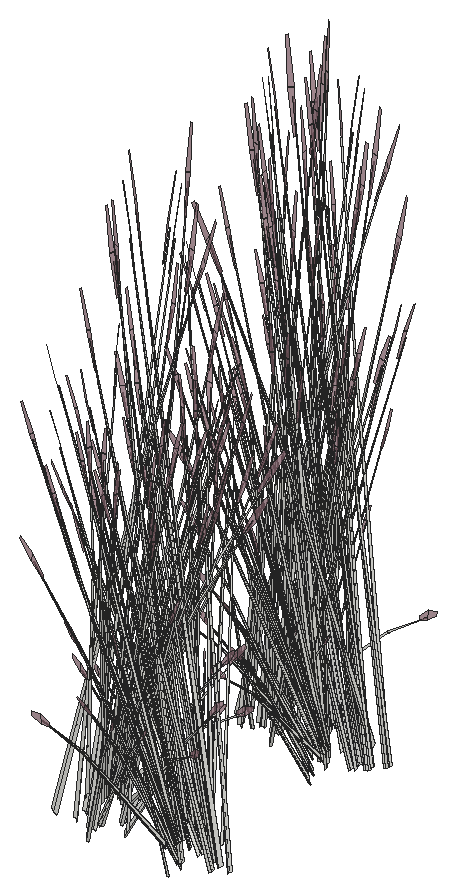
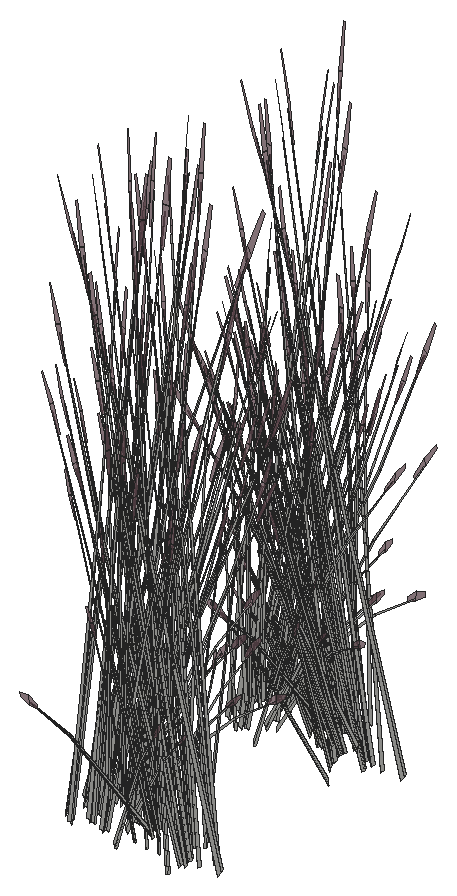
# SketchUp Ruby script. Lengths in inches.
U = 1.inch
M = Sketchup.active_model
def pt(a) = Geom::Point3d.new(a.map { |v| v * U })
def face(e, loops, mat)
  f = e.add_face(loops[0].map { |a| pt(a) })
  loops[1..].each { |l| e.add_face(l.map { |a| pt(a) }).erase! }
  f.material = f.back_material = mat if mat
  f
end
# faces: each face lists its corners as indices into pts; further lists are holes
def faces(e, pts, list, mat = nil) = list.each { |f| face(e, (f[0].is_a?(Array) ? f : [f]).map { |l| l.map { |i| pts[i] } }, mat) }
# xy, xz, yz: faces in a plane at the given z, y or x. An outline is a flat list of corners, or four numbers for a rectangle; further outlines are holes
def ring(l) = l.size == 4 ? [[l[0], l[1]], [l[2], l[1]], [l[2], l[3]], [l[0], l[3]]] : l.each_slice(2).to_a
def flat(e, list, mat, &to3) = list.each { |f| face(e, (f[0].is_a?(Array) ? f : [f]).map { |l| ring(l).map { |u, v| to3.(u, v) } }, mat) }
def xy(e, z, list, mat = nil) = flat(e, list, mat) { |x, y| [x, y, z] }
def xz(e, y, list, mat = nil) = flat(e, list, mat) { |x, z| [x, y, z] }
def yz(e, x, list, mat = nil) = flat(e, list, mat) { |y, z| [x, y, z] }
def lines(e, pts, list) = list.each { |a, b| e.add_line(pt(pts[a]), pt(pts[b])) }
# prism: a flat outline (further loops are holes) pulled along v
def prism(e, loops, v, mat = nil)
  f = face(e, loops, mat); d = Geom::Vector3d.new(v.map { |x| x * U })
  f.pushpull(f.normal.samedirection?(d) ? d.length : -d.length)
end
def box(e, o, s, mat = nil) = prism(e, [[o, [o[0] + s[0], o[1], o[2]], [o[0] + s[0], o[1] + s[1], o[2]], [o[0], o[1] + s[1], o[2]]]], [0, 0, s[2]], mat)
def at(x, y, z, deg = 0) = Geom::Transformation.translation(pt([x, y, z])) * Geom::Transformation.rotation(ORIGIN, Z_AXIS, deg.degrees)
def axes(o, x, y, z) = Geom::Transformation.new([*x, 0, *y, 0, *z, 0, *pt(o).to_a, 1])
def part(name) = M.definitions.add(name)
# library, detail: a bought-in or finely detailed component or shape, given as its bounding box
def library(name, o, s) = part(name).tap { |d| box(d.entities, o, s) }
def detail(e, o, s) = box(e.add_group.entities, o, s)
def put(e, d, t, mat = nil) = e.add_instance(d, t).tap { |i| i.material = mat if mat }
def group(e, t, mat = nil) = e.add_group.tap { |g| g.transformation = t; g.material = mat if mat }.entities
root = M.entities
M.materials.add("LightPink_Translucent").color = [144, 107, 117]
M.materials["LightPink_Translucent"].alpha = 0.75
c1 = part("blade")
p = [[2.15,0.21,22],[0,0.17,0],[0.09,0.45,0],[2.18,0.31,22],[2.29,0.31,22],[0.38,0.45,0],
  [2.48,0.24,33],[2.49,0.24,33],[2.48,0.22,33]]
faces(c1.entities,p,[[0,1,2,3],[4,5,2,3],[6,3,4,7],[8,0,3,6]])
c2 = part("seeds")
p = [[0.3,-0.1,1.38],[-0.01,-0.03,1.59],[-0.01,-0.03,0.03],[0.14,-0.07,-0.07],[0.29,-0.03,3],[0.15,0.01,3.11]]
faces(c2.entities,p,[[0,1,2,3],[1,0,4,5]],"LightPink_Translucent")
c3 = part("blade with seeds")
put(c3.entities,c1,at(0,0,0))
put(c3.entities,c2,axes([2.4,0.25,30.99],[1.5799,-0.05474,1.17369],[-0.12525,1.92788,0.29478],[-0.07173,-0.02425,1.56792]))
put(root,c3,axes([504.82,142.39,3.91],[-0.16348,-0.00431,1.74944],[-0.52047,0.43131,-0.27667],[-0.2777,-0.08813,0.14031]))
put(root,c3,axes([506.71,143.05,4.24],[0.11735,0.49217,0.35414],[-0.67083,0.12996,-0.4572],[-0.18018,-0.14104,0.87481]))
put(root,c3,axes([504.7,143.37,4.29],[0.62747,-0.45094,0.53763],[0.54116,0.47889,0.4433],[-0.29439,-0.08318,1.11249]))
put(root,c3,axes([495.97,144.28,0.6875],[-0.11372,-0.04814,1.76342],[-0.29211,-0.53779,-0.26939],[0.19706,-0.14594,0.30037]))
put(root,c3,axes([495.33,144.6,3.93],[0.54105,0.41691,0.48003],[-0.57458,0.35956,0.3958],[0.0998,-0.1956,0.9933]))
put(root,c3,axes([504.98,143.37,3.92],[0.03826,-0.46465,0.0643],[0.57772,0.01274,0.50621],[-0.2213,-0.04862,0.77189]))
put(root,c3,axes([504.76,143.51,3.72],[-0.43232,-0.38257,-0.35414],[0.49364,-0.36215,0.4572],[-0.25081,-0.0551,0.87481]))
put(root,c3,axes([495.97,145.8,4.17],[0.39688,-0.48213,-0.71045],[0.69548,0.34264,0.08574],[0.23697,-0.17468,1.00501]))
put(root,c3,axes([495.95,145.57,3.875],[-0.19519,-0.55794,-0.51099],[0.73919,-0.0976,-0.3958],[0.21183,-0.14986,0.97773]))
put(root,c3,axes([504.81,142.86,1.32],[-0.21918,0.49894,-0.03893],[-0.6746,-0.15348,-0.17649],[-0.10242,-0.08161,0.58215]))
put(root,c3,axes([504.45,145.14,1.57],[-0.95008,0,0],[0,-0.68292,-0.51607],[0,-0.15554,1.63711]))
put(root,c3,axes([504.61,143.92,1.78],[0.14835,0.17012,1.43002],[-0.34183,0.46242,-0.30754],[-0.351,-0.11053,0.61141]))
put(root,c3,axes([496.3,145.97,4.23],[-0.70283,-0.33692,-0.1216],[0.40491,-0.48793,-0.67495],[0.19857,-0.16961,1.02557]))
put(root,c3,axes([505.22,143.77,4.17],[-0.75952,-0.01471,-0.71045],[0.05101,-0.61953,0.08574],[-0.32177,-0.06538,1.00501]))
put(root,c3,axes([496.55,145.35,1.78],[-0.27143,-0.0181,1.43002],[-0.27808,-0.48551,-0.30754],[0.33346,-0.13735,0.61141]))
put(root,c3,axes([498.03,145.82,3.9],[-0.09924,-0.00464,1.77383],[-0.4121,-0.49725,-0.16761],[0.1655,-0.1635,0.31391]))
put(root,c3,axes([493.17,145.55,1.25],[0.51177,-0.45928,-0.62353],[0.63575,0.41646,-0.16365],[0.20507,-0.11457,1.37633]))
put(root,c3,axes([496.86,144.46,1.96],[-0.25308,0.31105,1.1486],[-0.21753,-0.4179,0.84392],[0.20902,-0.10472,0.25299]))
put(root,c3,axes([504.1875,142.76,3.9],[0.05633,0.06098,1.77383],[-0.27155,0.54815,-0.16761],[-0.27501,0.00397,0.31391]))
put(root,c3,axes([496.5,145.63,3.72],[0.66138,-0.08733,-0.35414],[0.17464,0.49921,0.4572],[0.18953,-0.13408,0.87481]))
put(root,c3,axes([504.97,143.89,3.875],[-0.55171,0.40476,-0.51099],[-0.48318,-0.42758,-0.3958],[-0.28031,-0.06159,0.97773]))
put(root,c3,axes([505.375,143.71,4.24],[0.43232,0.38257,0.35414],[-0.49364,0.36215,-0.4572],[-0.25081,-0.0551,0.87481]))
put(root,c3,axes([503.72,144.43,1.96],[0.48508,-0.04372,1.1486],[-0.3077,0.38525,0.84392],[-0.23971,-0.05779,0.25299]))
put(root,c3,axes([495.96,145.92,4.24],[-0.66138,0.08733,0.35414],[-0.17464,-0.49921,-0.4572],[0.18953,-0.13408,0.87481]))
put(root,c3,axes([505.26,143.47,4.23],[-0.04068,0.62141,-0.1216],[-0.77029,-0.01698,-0.67495],[-0.29667,-0.04317,1.02557]))
put(root,c3,axes([496.56,145.85,3.92],[0.52161,0.25698,0.0643],[-0.30368,0.36595,0.50621],[0.16723,-0.11831,0.77189]))
put(root,c3,axes([496.41,145.74,3.93],[0.18844,0.56237,0.48003],[-0.73919,0.0976,0.3958],[0.21785,-0.13226,0.9933]))
put(root,c3,axes([498.4,146.42,3.91],[0.10543,-0.09307,1.74944],[-0.13495,-0.57092,-0.27667],[0.26455,-0.10825,0.14031]))
put(root,c3,axes([506.62,145.93,1.25],[-0.79037,-0.10018,-0.62353],[0.16679,-0.61794,-0.16365],[-0.23587,-0.07488,1.37633]))
put(root,c3,axes([504.15,144.78,3.93],[0.21466,-0.55714,0.48003],[0.70573,0.19051,0.3958],[-0.27753,0.03348,0.9933]))
put(root,c3,axes([504.09,144.63,3.92],[-0.27906,-0.41663,0.0643],[0.50888,-0.20393,0.50621],[-0.22432,0.04024,0.77189]))
put(root,c3,axes([504.08,145.06,0.6875],[0.01927,0.0963,1.76342],[-0.38846,0.5029,-0.26939],[-0.27592,-0.02535,0.30037]))
put(root,c3,axes([505.78,146.875,1.22],[-0.17848,-0.53243,-0.30978],[0.70886,-0.15119,0.30978],[-0.1429,-0.0614,1.38974]))
put(root,c3,axes([496.33,147.29,4.23],[-0.38229,-0.5533,-0.1216],[0.6785,-0.2719,-0.67495],[0.28593,-0.073,1.02557]))
put(root,c3,axes([496.29,146.81,3.875],[0.20584,-0.55581,-0.51099],[0.70573,0.19051,-0.3958],[0.28414,-0.05097,0.97773]))
put(root,c3,axes([495.18,144.55,1.57],[0.47504,-0.61229,0],[0.79476,0.34146,-0.51607],[0.18101,0.07777,1.63711]))
put(root,c3,axes([505.58,147.1,1.21],[-0.7111,-0.30552,-0.49651],[0.42504,-0.54784,0],[-0.16196,-0.06958,1.57504]))
put(root,c3,axes([504,144.84,3.72],[-0.63144,-0.17046,-0.35414],[0.18417,-0.49731,0.4572],[-0.25423,0.0456,0.87481]))
put(root,c3,axes([497.05,146.97,1.17],[-0.48937,0.07333,1.41583],[-0.07789,-0.58369,0.08104],[0.34275,-0.08835,0.80566]))
put(root,c3,axes([497.9375,146.45,1.45],[-0.47106,-0.39072,-0.06488],[0.51591,-0.35801,-0.29416],[0.14618,-0.02521,0.97024]))
put(root,c3,axes([507.52,146.02,1.86],[-0.76714,0.40567,-0.29095],[-0.51013,-0.57321,-0.50002],[-0.18927,-0.05821,1.59708]))
put(root,c3,axes([496.16,147.01,4.17],[0.66765,-0.26986,-0.71045],[0.37208,0.55551,0.08574],[0.32259,-0.0631,1.00501]))
put(root,c3,axes([496.0625,147.12,4.24],[-0.63144,-0.17046,0.35414],[0.18417,-0.49731,-0.4572],[0.25423,-0.0456,0.87481]))
put(root,c3,axes([504.67,144.79,4.24],[0.63144,0.17046,0.35414],[-0.18417,0.49731,-0.4572],[-0.25423,0.0456,0.87481]))
put(root,c3,axes([491.74,145.63,0.79],[-0.74787,0.24464,1.28929],[-0.23804,-0.70192,0.50096],[0.45924,0.01168,1.46642]))
put(root,c3,axes([497.58,146.59,0.6875],[-0.03971,-0.09277,1.76342],[0.27541,-0.54264,-0.26939],[0.27782,-0.00781,0.30037]))
put(root,c3,axes([505.92,144.76,2.53],[0.21597,-0.08839,1.77064],[0.07448,0.61717,0.13857],[-0.4678,0.08189,0.63284]))
put(root,c3,axes([493.68,145.99,1.86],[0.76714,-0.40567,-0.29095],[0.51013,0.57321,-0.50002],[0.18927,0.05821,1.59708]))
put(root,c3,axes([496.73,147.0625,3.72],[0.63144,0.17046,-0.35414],[-0.18417,0.49731,0.4572],[0.25423,-0.0456,0.87481]))
put(root,c3,axes([495.61,144.92,1.21],[0.7111,0.30552,-0.49651],[-0.42504,0.54784,0],[0.16196,0.06958,1.57504]))
put(root,c3,axes([503.6,145.17,3.91],[-0.12407,0.07933,1.74944],[0.01055,0.57963,-0.27667],[-0.2844,0.07538,0.14031]))
put(root,c3,axes([504.43,145.09,3.875],[-0.20584,0.55581,-0.51099],[-0.70573,-0.19051,-0.3958],[-0.28414,0.05097,0.97773]))
put(root,c3,axes([504.4,144.62,4.23],[0.38229,0.5533,-0.1216],[-0.6785,0.2719,-0.67495],[-0.28593,0.073,1.02557]))
put(root,c3,axes([506.02,147.47,1.57],[-0.47504,0.61229,0],[-0.79476,-0.34146,-0.51607],[-0.18101,-0.07777,1.63711]))
put(root,c3,axes([495.01,146.45,3.07],[-0.31515,0.01384,1.71376],[0.20907,-0.5998,0.13857],[0.44912,0.0371,0.73262]))
put(root,c3,axes([495.41,145.14,1.22],[0.17848,0.53243,-0.30978],[-0.70886,0.15119,0.30978],[0.1429,0.0614,1.38974]))
put(root,c3,axes([496.63,147.27,3.92],[0.27906,0.41663,0.0643],[-0.50888,0.20393,0.50621],[0.22432,-0.04024,0.77189]))
put(root,c3,axes([496.58,147.125,3.93],[-0.21466,0.55714,0.48003],[-0.70573,-0.19051,0.3958],[0.27753,-0.03348,0.9933]))
put(root,c3,axes([494.57,146.09,1.25],[0.79037,0.10018,-0.62353],[-0.16679,0.61794,-0.16365],[0.23587,0.07488,1.37633]))
put(root,c3,axes([504.32,146.17,3.93],[-0.18844,-0.56237,0.48003],[0.73919,-0.0976,0.3958],[-0.21785,0.13226,0.9933]))
put(root,c3,axes([498.07,147.16,1.96],[-0.46945,0.10088,1.1486],[0.22097,-0.4169,0.84392],[0.24904,0.02853,0.25299]))
put(root,c3,axes([504.17,146.06,3.92],[-0.52161,-0.25698,0.0643],[0.30368,-0.36595,0.50621],[-0.16723,0.11831,0.77189]))
put(root,c3,axes([497.85,148.93,3.9],[-0.0687,-0.05349,1.77383],[0.15029,-0.57341,-0.16761],[0.27062,-0.03664,0.31391]))
put(root,c3,axes([497.25,148.45,3.12],[-0.14542,-0.51365,-0.03492],[0.68734,-0.11809,-0.15832],[0.14353,0.03256,0.52218]))
put(root,c3,axes([495.47,148.44,4.23],[0.04068,-0.62141,-0.1216],[0.77029,0.01698,-0.67495],[0.29667,0.04317,1.02557]))
put(root,c3,axes([504.77,145.98,4.24],[0.66138,-0.08733,0.35414],[0.17464,0.49921,-0.4572],[-0.18953,0.13408,0.87481]))
put(root,c3,axes([502.22,145.76,3.9],[0.09697,0.01639,1.77383],[0.29997,0.53988,-0.16761],[-0.1985,0.1417,0.31391]))
put(root,c3,axes([495.35,148.19,4.24],[-0.43232,-0.38257,0.35414],[0.49364,-0.36215,-0.4572],[0.25081,0.0551,0.87481]))
put(root,c3,axes([503.04,147.47,1.96],[0.31665,-0.27694,1.1486],[0.12495,0.43841,0.84392],[-0.22883,0.0785,0.25299]))
put(root,c3,axes([504.23,146.28,3.72],[-0.66138,0.08733,-0.35414],[-0.17464,-0.49921,0.4572],[-0.18953,0.13408,0.87481]))
put(root,c3,axes([496.14,148.0625,3.91],[0.16299,-0.01033,1.74944],[0.44707,-0.47471,-0.27667],[0.28992,0.06266,0.14031]))
put(root,c3,axes([503.27,147.4,4.84],[0.67048,0.16311,-0.06488],[-0.20625,0.50201,-0.29416],[-0.10966,0.07622,0.97024]))
put(root,c3,axes([508.03,146.47,1.25],[-0.51177,0.45928,-0.62353],[-0.63575,-0.41646,-0.16365],[-0.20507,0.11457,1.37633]))
put(root,c3,axes([495.51,148.14,4.17],[0.75952,0.01471,-0.71045],[-0.05101,0.61953,0.08574],[0.32177,0.06538,1.00501]))
put(root,c3,axes([504.43,145.93,4.23],[0.70283,0.33692,-0.1216],[-0.40491,0.48793,-0.67495],[-0.19857,0.16961,1.02557]))
put(root,c3,axes([505.375,145.78,3.07],[0.18977,-0.18775,1.71376],[0.47917,0.50677,0.13857],[-0.32866,0.23079,0.73262]))
put(root,c3,axes([496.75,146.88,1.57],[0.95008,0,0],[0,0.68292,-0.51607],[0,0.15554,1.63711]))
put(root,c3,axes([504.78,146.33,3.875],[0.19519,0.55794,-0.51099],[-0.73919,0.0976,-0.3958],[-0.21183,0.14986,0.97773]))
put(root,c3,axes([495.96,148.39,3.72],[0.43232,0.38257,-0.35414],[-0.49364,0.36215,0.4572],[0.25081,0.0551,0.87481]))
put(root,c3,axes([495.74,148.54,3.92],[-0.03826,0.46465,0.0643],[-0.57772,-0.01274,0.50621],[0.2213,0.04862,0.77189]))
put(root,c3,axes([505.2,147.27,3.92],[-0.62439,-0.02847,0.0643],[0.01712,-0.42991,0.50621],[-0.06534,0.16468,0.77189]))
put(root,c3,axes([503.87,147.76,0.6875],[0.10192,0.06105,1.76342],[0.17281,0.56562,-0.26939],[-0.22588,0.12062,0.30037]))
put(root,c3,axes([505.4,147.31,3.93],[-0.54105,-0.41691,0.48003],[0.57458,-0.35956,0.3958],[-0.0998,0.1956,0.9933]))
put(root,c3,axes([495.8,148.39,3.93],[-0.56024,0.40262,0.48003],[-0.48318,-0.42758,0.3958],[0.26285,0.07427,0.9933]))
put(root,c3,axes([494.41,147.41,3.07],[-0.28223,-0.10528,1.71376],[0.58406,-0.44165,0.13857],[0.36402,0.19924,0.73262]))
put(root,c3,axes([505.23,146.25,3.07],[0.14147,-0.21002,1.71376],[0.59349,0.43464,0.13857],[-0.26773,0.27089,0.73262]))
put(root,c3,axes([493.95,149.11,4.23],[0.45276,-0.52302,-0.1216],[0.65568,0.30132,-0.67495],[0.22792,0.14777,1.02557]))
put(root,c3,axes([505.39,147.43,3.72],[-0.5141,0.32171,-0.35414],[-0.48666,-0.36734,0.4572],[-0.07405,0.18664,0.87481]))
put(root,c3,axes([503.62,147.34,3.91],[-0.01889,0.12092,1.74944],[0.53598,0.42065,-0.27667],[-0.14032,0.19892,0.14031]))
put(root,c3,axes([495.58,149.26,0.6875],[0.05536,-0.08822,1.76342],[0.69692,-0.25981,-0.26939],[0.21129,0.13447,0.30037]))
put(root,c3,axes([494.49,148.85,3.875],[0.74975,-0.14525,-0.51099],[0.13115,0.55007,-0.3958],[0.20138,0.15763,0.97773]))
put(root,c3,axes([495.52,149.41,1.86],[-0.48723,-0.01916,1.0506],[0.32177,-0.40701,0.58006],[0.19248,0.1446,0.8241]))
put(root,c3,axes([505.15,148.36,1.78],[0.23977,-0.09639,1.43002],[0.59198,0.29065,-0.30754],[-0.1762,0.25149,0.61141]))
put(root,c3,axes([504.4,161.67,3.07],[0.17368,0.19618,1.71376],[-0.80256,0.16516,0.13857],[-0.18139,-0.30799,0.73262]))
put(root,c3,axes([505.72,160.37,3.91],[-0.11621,-0.08567,1.74944],[-0.77555,0.05431,-0.27667],[-0.12378,-0.20491,0.14031]))
put(root,c3,axes([504.18,161.15,1.78],[-0.04601,0.19989,1.43002],[-0.67263,0.16733,-0.30754],[-0.15723,-0.25836,0.61141]))
put(root,c3,axes([504.93,160.09,3.9],[-0.01417,0.07324,1.77383],[-0.6991,0.2658,-0.16761],[-0.20573,-0.13587,0.31391]))
put(root,c3,axes([504.77,161.39,4.29],[0.84639,-0.15705,0.53763],[0.14689,0.61608,0.4433],[-0.19906,-0.18157,1.11249]))
put(root,c3,axes([503.95,160.83,1.96],[0.39634,0.21267,1.1486],[-0.57721,0.12784,0.84392],[-0.1235,-0.16344,0.25299]))
put(root,c3,axes([504.9,161.96,4.17],[-0.64788,-0.29534,-0.71045],[0.46044,-0.51755,0.08574],[-0.23473,-0.17635,1.00501]))
put(root,c3,axes([504.68,161.57,3.72],[-0.11735,-0.49217,-0.35414],[0.67083,-0.12996,0.4572],[-0.18018,-0.14104,0.87481]))
put(root,c3,axes([504.97,161.52,3.92],[0.34533,-0.38816,0.0643],[0.49176,0.22599,0.50621],[-0.15898,-0.12445,0.77189]))
put(root,c3,axes([503.63,161.47,0.6875],[-0.0736,0.08049,1.76342],[-0.74378,0.17355,-0.26939],[-0.17968,-0.15788,0.30037]))
put(root,c3,axes([504.6,161.97,3.875],[-0.74975,0.14525,-0.51099],[-0.13115,-0.55007,-0.3958],[-0.20138,-0.15763,0.97773]))
put(root,c3,axes([505.125,161.48,4.62],[-0.50709,0.58578,-0.13619],[-0.73436,-0.33748,-0.75594],[-0.25527,-0.1655,1.14864]))
put(root,c3,axes([496.08,164.04,1.78],[-0.21597,0.12368,1.43002],[-0.64681,-0.21647,-0.30754],[0.1199,-0.26922,0.61141]))
put(root,c3,axes([503.18,161.3125,3.91],[-0.16348,-0.00431,1.74944],[-0.52047,0.43131,-0.27667],[-0.2777,-0.08813,0.14031]))
put(root,c3,axes([496.61,164.95,4.17],[0.01977,-0.56521,-0.71045],[0.83252,0.03796,0.08574],[0.08786,-0.23945,1.00501]))
put(root,c3,axes([497.77,164.07,3.91],[-0.00733,-0.12161,1.74944],[-0.61946,-0.35147,-0.27667],[0.09577,-0.21306,0.14031]))
put(root,c3,axes([495.67,164.67,3.07],[-0.14147,0.21002,1.71376],[-0.59349,-0.43464,0.13857],[0.26773,-0.27089,0.73262]))
put(root,c3,axes([506.45,165.3,2.52],[0.65659,0.2464,1.51261],[-0.64324,0.53082,0.59816],[-0.28812,-0.31461,1.26806]))
put(root,c3,axes([505.08,161.97,4.24],[0.11735,0.49217,0.35414],[-0.67083,0.12996,-0.4572],[-0.18018,-0.14104,0.87481]))
put(root,c3,axes([503.02,163.6,1.21],[0,-0.61104,-0.49651],[0.85008,0,0],[0,-0.13917,1.57504]))
put(root,c3,axes([503.0625,162.29,4.29],[0.62747,-0.45094,0.53763],[0.54116,0.47889,0.4433],[-0.29439,-0.08318,1.11249]))
put(root,c3,axes([503.35,162.29,3.92],[0.03826,-0.46465,0.0643],[0.57772,0.01274,0.50621],[-0.2213,-0.04862,0.77189]))
put(root,c3,axes([503.125,162.43,3.72],[-0.43232,-0.38257,-0.35414],[0.49364,-0.36215,0.4572],[-0.25081,-0.0551,0.87481]))
put(root,c3,axes([496.95,164.61,3.72],[0.5141,-0.32171,-0.35414],[0.48666,0.36734,0.4572],[0.07405,-0.18664,0.87481]))
put(root,c3,axes([503.17,161.78,1.32],[-0.21918,0.49894,-0.03893],[-0.6746,-0.15348,-0.17649],[-0.10242,-0.08161,0.58215]))
put(root,c3,axes([502.81,164.06,1.57],[-0.95008,0,0],[0,-0.68292,-0.51607],[0,-0.15554,1.63711]))
put(root,c3,axes([497.59,164.42,0.6875],[-0.11372,-0.04814,1.76342],[-0.29211,-0.53779,-0.26939],[0.19706,-0.14594,0.30037]))
put(root,c3,axes([496.95,164.74,3.93],[0.54105,0.41691,0.48003],[-0.57458,0.35956,0.3958],[0.0998,-0.1956,0.9933]))
put(root,c3,axes([503.54,163.88,1.52],[-0.70674,0.51372,0.30756],[-0.70717,-0.50832,-0.36492],[-0.02468,-0.14589,1.64885]))
put(root,c3,axes([497.15,164.78,3.92],[0.62439,0.02847,0.0643],[-0.01712,0.42991,0.50621],[0.06534,-0.16468,0.77189]))
put(root,c3,axes([505.46,164.95,1.63],[0.20138,-0.72405,-0.23429],[0.95485,0.12621,0.51271],[-0.16685,-0.09999,1.5644]))
put(root,c3,axes([497.59,165.94,4.17],[0.39688,-0.48213,-0.71045],[0.69548,0.34264,0.08574],[0.23697,-0.17468,1.00501]))
put(root,c3,axes([497.57,165.71,3.875],[-0.19519,-0.55794,-0.51099],[0.73919,-0.0976,-0.3958],[0.21183,-0.14986,0.97773]))
put(root,c3,axes([503.74,162.63,4.24],[0.43232,0.38257,0.35414],[-0.49364,0.36215,-0.4572],[-0.25081,-0.0551,0.87481]))
put(root,c3,axes([502.09,163.35,1.96],[0.48508,-0.04372,1.1486],[-0.3077,0.38525,0.84392],[-0.23971,-0.05779,0.25299]))
put(root,c3,axes([497.92,166.11,4.23],[-0.70283,-0.33692,-0.1216],[0.40491,-0.48793,-0.67495],[0.19857,-0.16961,1.02557]))
put(root,c3,axes([503.62,162.39,4.23],[-0.04068,0.62141,-0.1216],[-0.77029,-0.01698,-0.67495],[-0.29667,-0.04317,1.02557]))
put(root,c3,axes([503.38,164.16,1.67],[0,0.61104,0.49651],[-0.85008,0,0],[0,-0.13917,1.57504]))
put(root,c3,axes([505.39,164.66,1.4],[-0.45644,-0.51287,-0.44739],[0.69137,-0.36116,0.21531],[-0.14771,-0.06346,1.43643]))
put(root,c3,axes([493.95,164.4375,1.21],[0.7111,-0.30552,-0.49651],[0.42504,0.54784,0],[0.16196,-0.06958,1.57504]))
put(root,c3,axes([499.65,165.96,3.9],[-0.09924,-0.00464,1.77383],[-0.4121,-0.49725,-0.16761],[0.1655,-0.1635,0.31391]))
put(root,c3,axes([494.79,165.69,1.25],[0.51177,-0.45928,-0.62353],[0.63575,0.41646,-0.16365],[0.20507,-0.11457,1.37633]))
put(root,c3,axes([498.48,164.6,1.96],[-0.25308,0.31105,1.1486],[-0.21753,-0.4179,0.84392],[0.20902,-0.10472,0.25299]))
put(root,c3,axes([504.98,164.85,1.25],[-0.79037,-0.10018,-0.62353],[0.16679,-0.61794,-0.16365],[-0.23587,-0.07488,1.37633]))
put(root,c3,axes([498.12,165.77,3.72],[0.66138,-0.08733,-0.35414],[0.17464,0.49921,0.4572],[0.18953,-0.13408,0.87481]))
put(root,c3,axes([502.51,163.7,3.93],[0.21466,-0.55714,0.48003],[0.70573,0.19051,0.3958],[-0.27753,0.03348,0.9933]))
put(root,c3,axes([502.46,163.55,3.92],[-0.27906,-0.41663,0.0643],[0.50888,-0.20393,0.50621],[-0.22432,0.04024,0.77189]))
put(root,c3,axes([497.58,166.0625,4.24],[-0.66138,0.08733,0.35414],[-0.17464,-0.49921,-0.4572],[0.18953,-0.13408,0.87481]))
put(root,c3,axes([504.14,165.79,1.22],[-0.17848,-0.53243,-0.30978],[0.70886,-0.15119,0.30978],[-0.1429,-0.0614,1.38974]))
put(root,c3,axes([494.11,164.68,1.22],[0.70886,0.15119,-0.30978],[-0.17848,0.53243,0.30978],[0.1429,-0.0614,1.38974]))
put(root,c3,axes([503.94,166.02,1.21],[-0.7111,-0.30552,-0.49651],[0.42504,-0.54784,0],[-0.16196,-0.06958,1.57504]))
put(root,c3,axes([498.18,165.98,3.92],[0.52161,0.25698,0.0643],[-0.30368,0.36595,0.50621],[0.16723,-0.11831,0.77189]))
put(root,c3,axes([498.03,165.875,3.93],[0.18844,0.56237,0.48003],[-0.73919,0.0976,0.3958],[0.21785,-0.13226,0.9933]))
put(root,c3,axes([505.88,164.94,1.86],[-0.76714,0.40567,-0.29095],[-0.51013,-0.57321,-0.50002],[-0.18927,-0.05821,1.59708]))
put(root,c3,axes([505.81,165.12,1.81],[-0.14658,0.54532,0.1448],[-0.71613,-0.09466,-0.41347],[-0.13033,-0.05599,1.26744]))
put(root,c3,axes([503.03,163.71,4.24],[0.63144,0.17046,0.35414],[-0.18417,0.49731,-0.4572],[-0.25423,0.0456,0.87481]))
put(root,c3,axes([497.95,167.42,4.23],[-0.38229,-0.5533,-0.1216],[0.6785,-0.2719,-0.67495],[0.28593,-0.073,1.02557]))
put(root,c3,axes([497.91,166.95,3.875],[0.20584,-0.55581,-0.51099],[0.70573,0.19051,-0.3958],[0.28414,-0.05097,0.97773]))
put(root,c3,axes([496.8,164.69,1.57],[0.47504,-0.61229,0],[0.79476,0.34146,-0.51607],[0.18101,0.07777,1.63711]))
put(root,c3,axes([506.74,165.13,1.66],[-0.74193,-0.49181,-0.25192],[0.6243,-0.55226,0.5513],[-0.19979,0.05753,1.68216]))
put(root,c3,axes([504.79,166.07,1.67],[0.7111,0.30552,0.49651],[-0.42504,0.54784,0],[-0.16196,-0.06958,1.57504]))
put(root,c3,axes([499.56,166.59,1.45],[-0.47106,-0.39072,-0.06488],[0.51591,-0.35801,-0.29416],[0.14618,-0.02521,0.97024]))
put(root,c3,axes([496.39,165.01,1.67],[-0.7111,-0.30552,0.49651],[0.42504,-0.54784,0],[0.16196,0.06958,1.57504]))
put(root,c3,axes([502.76,163.54,4.23],[0.38229,0.5533,-0.1216],[-0.6785,0.2719,-0.67495],[-0.28593,0.073,1.02557]))
put(root,c3,axes([504.38,166.39,1.57],[-0.47504,0.61229,0],[-0.79476,-0.34146,-0.51607],[-0.18101,-0.07777,1.63711]))
put(root,c3,axes([497.68,167.26,4.24],[-0.63144,-0.17046,0.35414],[0.18417,-0.49731,-0.4572],[0.25423,-0.0456,0.87481]))
put(root,c3,axes([506.36,165.03,1.4],[-0.82508,0.03772,-0.44739],[-0.07462,-0.62614,0.21531],[-0.14771,0.06346,1.43643]))
put(root,c3,axes([493.36,165.77,0.79],[-0.74787,0.24464,1.28929],[-0.23804,-0.70192,0.50096],[0.45924,0.01168,1.46642]))
put(root,c3,axes([495.37,165.96,1.81],[0.14658,-0.54532,0.1448],[0.71613,0.09466,-0.41347],[0.13033,0.05599,1.26744]))
put(root,c3,axes([507.28,166.48,1.39],[-0.46912,-0.61443,-0.05142],[0.79476,-0.34146,0.51607],[-0.19584,0.0585,1.6363]))
put(root,c3,axes([502.68,165.09,3.93],[-0.18844,-0.56237,0.48003],[0.73919,-0.0976,0.3958],[-0.21785,0.13226,0.9933]))
put(root,c3,axes([502.53,164.98,3.92],[-0.52161,-0.25698,0.0643],[0.30368,-0.36595,0.50621],[-0.16723,0.11831,0.77189]))
put(root,c3,axes([495.3,166.13,1.86],[0.76714,-0.40567,-0.29095],[0.51013,0.57321,-0.50002],[0.18927,0.05821,1.59708]))
put(root,c3,axes([497.23,165.05,1.21],[0.7111,0.30552,-0.49651],[-0.42504,0.54784,0],[0.16196,0.06958,1.57504]))
put(root,c3,axes([507.0625,166.4,1.22],[-0.70886,-0.15119,-0.30978],[0.17848,-0.53243,0.30978],[-0.1429,0.0614,1.38974]))
put(root,c3,axes([497.03,165.28,1.22],[0.17848,0.53243,-0.30978],[-0.70886,0.15119,0.30978],[0.1429,0.0614,1.38974]))
put(root,c3,axes([503.13,164.9,4.24],[0.66138,-0.08733,0.35414],[0.17464,0.49921,-0.4572],[-0.18953,0.13408,0.87481]))
put(root,c3,axes([498.25,167.41,3.92],[0.27906,0.41663,0.0643],[-0.50888,0.20393,0.50621],[0.22432,-0.04024,0.77189]))
put(root,c3,axes([498.2,167.26,3.93],[-0.21466,0.55714,0.48003],[-0.70573,-0.19051,0.3958],[0.27753,-0.03348,0.9933]))
put(root,c3,axes([501.4,166.39,1.96],[0.31665,-0.27694,1.1486],[0.12495,0.43841,0.84392],[-0.22883,0.0785,0.25299]))
put(root,c3,axes([495.77,168.2,1.38],[0.79769,-0.20732,-0.19198],[0.2803,0.59721,0.00008],[0.08805,-0.02292,1.73897]))
put(root,c3,axes([502.59,165.2,3.72],[-0.66138,0.08733,-0.35414],[-0.17464,-0.49921,0.4572],[-0.18953,0.13408,0.87481]))
put(root,c3,axes([496.19,166.22,1.25],[0.79037,0.10018,-0.62353],[-0.16679,0.61794,-0.16365],[0.23587,0.07488,1.37633]))
put(root,c3,axes([501.63,166.32,4.84],[0.67048,0.16311,-0.06488],[-0.20625,0.50201,-0.29416],[-0.10966,0.07622,0.97024]))
put(root,c3,axes([506.39,165.39,1.25],[-0.51177,0.45928,-0.62353],[-0.63575,-0.41646,-0.16365],[-0.20507,0.11457,1.37633]))
put(root,c3,axes([507.23,166.64,1.21],[-0.7111,0.30552,-0.49651],[-0.42504,-0.54784,0],[-0.16196,0.06958,1.57504]))
put(root,c3,axes([495.78,166.42,1.4],[0.45644,0.51287,-0.44739],[-0.69137,0.36116,0.21531],[0.14771,0.06346,1.43643]))
put(root,c3,axes([498.87,168.59,3.12],[-0.14542,-0.51365,-0.03492],[0.68734,-0.11809,-0.15832],[0.14353,0.03256,0.52218]))
put(root,c3,axes([497.09,168.57,4.23],[0.04068,-0.62141,-0.1216],[0.77029,0.01698,-0.67495],[0.29667,0.04317,1.02557]))
put(root,c3,axes([502.79,164.85,4.23],[0.70283,0.33692,-0.1216],[-0.40491,0.48793,-0.67495],[-0.19857,0.16961,1.02557]))
put(root,c3,axes([497.79,166.91,1.67],[0,-0.61104,0.49651],[0.85008,0,0],[0,0.13917,1.57504]))
put(root,c3,axes([496.97,168.33,4.24],[-0.43232,-0.38257,0.35414],[0.49364,-0.36215,-0.4572],[0.25081,0.0551,0.87481]))
put(root,c3,axes([503.74,164.7,3.07],[0.18977,-0.18775,1.71376],[0.47917,0.50677,0.13857],[-0.32866,0.23079,0.73262]))
put(root,c3,axes([503.14,165.25,3.875],[0.19519,0.55794,-0.51099],[-0.73919,0.0976,-0.3958],[-0.21183,0.14986,0.97773]))
put(root,c3,axes([503.56,166.1875,3.92],[-0.62439,-0.02847,0.0643],[0.01712,-0.42991,0.50621],[-0.06534,0.16468,0.77189]))
put(root,c3,axes([502.23,166.68,0.6875],[0.10192,0.06105,1.76342],[0.17281,0.56562,-0.26939],[-0.22588,0.12062,0.30037]))
put(root,c3,axes([503.76,166.23,3.93],[-0.54105,-0.41691,0.48003],[0.57458,-0.35956,0.3958],[-0.0998,0.1956,0.9933]))
put(root,c3,axes([497.76,168.2,3.91],[0.16299,-0.01033,1.74944],[0.44707,-0.47471,-0.27667],[0.28992,0.06266,0.14031]))
